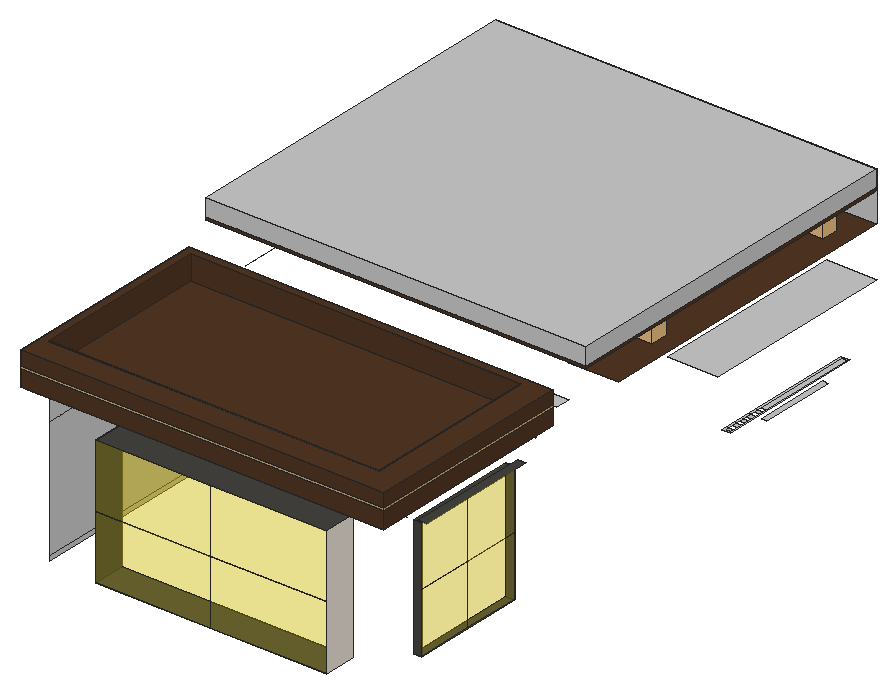
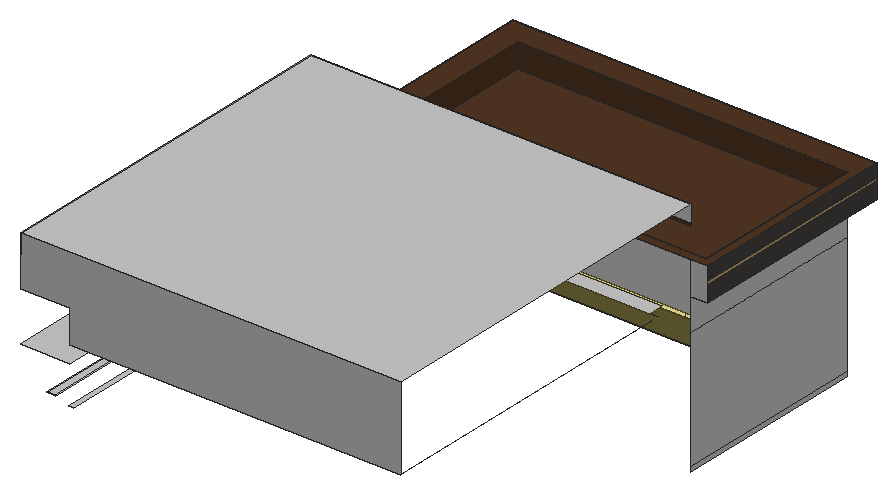
# SketchUp Ruby script. Lengths in inches.
U = 1.inch
M = Sketchup.active_model
def pt(a) = Geom::Point3d.new(a.map { |v| v * U })
def face(e, loops, mat)
  f = e.add_face(loops[0].map { |a| pt(a) })
  loops[1..].each { |l| e.add_face(l.map { |a| pt(a) }).erase! }
  f.material = f.back_material = mat if mat
  f
end
# faces: each face lists its corners as indices into pts; further lists are holes
def faces(e, pts, list, mat = nil) = list.each { |f| face(e, (f[0].is_a?(Array) ? f : [f]).map { |l| l.map { |i| pts[i] } }, mat) }
# xy, xz, yz: faces in a plane at the given z, y or x. An outline is a flat list of corners, or four numbers for a rectangle; further outlines are holes
def ring(l) = l.size == 4 ? [[l[0], l[1]], [l[2], l[1]], [l[2], l[3]], [l[0], l[3]]] : l.each_slice(2).to_a
def flat(e, list, mat, &to3) = list.each { |f| face(e, (f[0].is_a?(Array) ? f : [f]).map { |l| ring(l).map { |u, v| to3.(u, v) } }, mat) }
def xy(e, z, list, mat = nil) = flat(e, list, mat) { |x, y| [x, y, z] }
def xz(e, y, list, mat = nil) = flat(e, list, mat) { |x, z| [x, y, z] }
def yz(e, x, list, mat = nil) = flat(e, list, mat) { |y, z| [x, y, z] }
def lines(e, pts, list) = list.each { |a, b| e.add_line(pt(pts[a]), pt(pts[b])) }
# prism: a flat outline (further loops are holes) pulled along v
def prism(e, loops, v, mat = nil)
  f = face(e, loops, mat); d = Geom::Vector3d.new(v.map { |x| x * U })
  f.pushpull(f.normal.samedirection?(d) ? d.length : -d.length)
end
def box(e, o, s, mat = nil) = prism(e, [[o, [o[0] + s[0], o[1], o[2]], [o[0] + s[0], o[1] + s[1], o[2]], [o[0], o[1] + s[1], o[2]]]], [0, 0, s[2]], mat)
def at(x, y, z, deg = 0) = Geom::Transformation.translation(pt([x, y, z])) * Geom::Transformation.rotation(ORIGIN, Z_AXIS, deg.degrees)
def axes(o, x, y, z) = Geom::Transformation.new([*x, 0, *y, 0, *z, 0, *pt(o).to_a, 1])
def part(name) = M.definitions.add(name)
# library, detail: a bought-in or finely detailed component or shape, given as its bounding box
def library(name, o, s) = part(name).tap { |d| box(d.entities, o, s) }
def detail(e, o, s) = box(e.add_group.entities, o, s)
def put(e, d, t, mat = nil) = e.add_instance(d, t).tap { |i| i.material = mat if mat }
def group(e, t, mat = nil) = e.add_group.tap { |g| g.transformation = t; g.material = mat if mat }.entities
root = M.entities
M.materials.add("Glass_Basic_01").color = [255, 228, 0]
M.materials["Glass_Basic_01"].alpha = 0.25
M.materials.add("Marble_01_1K").color = [230, 221, 211]
M.materials.add("Plywood_08_1K").color = [202, 166, 113]
M.materials.add("Wood_Planks_01_1K").color = [69, 67, 63]
M.materials.add("Wood_Veneer_15_1K").color = [81, 54, 35]
M.materials.add("[_0053_Ivory_]").color = [200, 200, 200]
c1 = library("Sphere Light\#3",[-4.91,-4.91,-4.91],[9.82,9.82,9.82])
c2 = library("Sphere Light\#2",[-4.71,-4.71,-4.71],[9.42,9.42,9.42])
c3 = library("Sphere Light\#1",[-6.34,-6.34,-6.34],[12.68,12.68,12.68])
c4 = library("Sphere Light",[-6.24,-6.24,-6.24],[12.48,12.48,12.48])
xy(root,267,[[410.51,98.15,578.51,122.15]],"Wood_Planks_01_1K")
xy(root,270,[[605.51,143.15,611.51,227.15]],"Wood_Planks_01_1K")
xy(root,318,[[643.1,411.95,647.1,467.15]],"[_0053_Ivory_]")
xy(root,330,[[[647.1,371.15,653.51,479.15],[648.1,372.15,652.51,478.15]],[648.1,372.15,652.51,375.42],[648.1,378.69,652.51,381.96],[648.1,385.24,652.51,388.51],[648.1,391.78,652.51,395.05],
  [648.1,398.33,652.51,401.6],[648.1,404.87,652.51,478.15]],"[_0053_Ivory_]")
xy(root,357,[[605.51,143.15,611.51,227.15]],"Wood_Planks_01_1K")
xy(root,360,[[410.51,98.15,578.51,122.15],[611.51,140.15,617.51,230.15]],"Wood_Planks_01_1K")
xy(root,372,[[386.51,122.15,605.51,239.15],[617.51,359.15,653.51,503.15]],"[_0053_Ivory_]")
xy(root,384,[[365.51,98.15,365.51,239.15,377.51,239.15,377.51,98.15,377.33,98.15,376.79,98.5625,375.34,99.16,373.79,99.37,372.23,99.16,370.79,98.5625,370.25,98.15]],"Wood_Planks_01_1K")
xy(root,384,[[365.51,86.15,365.51,98.15,370.25,98.15,369.55,97.61,368.59,96.37,367.99,94.92,367.79,93.37,367.99,91.8125,368.59,90.37,369.55,89.12,370.79,88.17,372.23,87.57,373.79,87.37,375.34,87.57,376.79,88.17,378.03,89.12,378.98,90.37,379.58,91.8125,379.79,93.37,379.58,94.92,378.98,96.37,378.03,97.61,377.33,98.15,618.11,98.15,617.41,97.61,616.46,96.37,615.86,94.92,615.65,93.37,615.86,91.8125,616.46,90.37,617.41,89.12,618.65,88.17,620.1,87.57,621.65,87.37,623.2,87.57,624.65,88.17,625.89,89.12,626.85,90.37,627.45,91.8125,627.65,93.37,627.45,94.92,626.85,96.37,625.89,97.61,625.19,98.15,629.51,98.15,629.51,86.15],[617.51,98.15,617.51,239.15,629.51,239.15,629.51,98.15,625.19,98.15,624.65,98.5625,623.2,99.16,621.65,99.37,620.1,99.16,618.65,98.5625,618.11,98.15]],"Wood_Veneer_15_1K")
xy(root,384,[[383.51,257.92,617.51,269.15]],"[_0053_Ivory_]")
xy(root,387,[[373.79,87.37,372.23,87.57,370.79,88.17,369.55,89.12,368.59,90.37,367.99,91.8125,367.79,93.37,367.99,94.92,368.59,96.37,369.55,97.61,370.25,98.15,370.79,98.5625,372.23,99.16,373.79,99.37,375.34,99.16,376.79,98.5625,377.33,98.15,378.03,97.61,378.98,96.37,379.58,94.92,379.79,93.37,379.58,91.8125,378.98,90.37,378.03,89.12,376.79,88.17,375.34,87.57],[621.65,87.37,620.1,87.57,618.65,88.17,617.41,89.12,616.46,90.37,615.86,91.8125,615.65,93.37,615.86,94.92,616.46,96.37,617.41,97.61,618.11,98.15,618.65,98.5625,620.1,99.16,621.65,99.37,623.2,99.16,624.65,98.5625,625.19,98.15,625.89,97.61,626.85,96.37,627.45,94.92,627.65,93.37,627.45,91.8125,626.85,90.37,625.89,89.12,624.65,88.17,623.2,87.57]],"Wood_Veneer_15_1K")
xy(root,390.44,[[371.51,104.15,611.51,233.15]],"Wood_Veneer_15_1K")
xy(root,408,[[[365.51,86.15,629.51,239.15],[371.51,104.15,611.51,233.15]],[[617.51,269.15,653.51,503.15],[633.43,316.8125,634.98,317.02,636.43,317.62,637.67,318.57,638.62,319.8125,639.22,321.26,639.43,322.8125,639.22,324.37,638.62,325.8125,637.67,327.06,636.43,328.01,634.98,328.61,633.43,328.8125,631.875,328.61,630.43,328.01,629.18,327.06,628.23,325.8125,627.63,324.37,627.43,322.8125,627.63,321.26,628.23,319.8125,629.18,318.57,630.43,317.62,631.875,317.02],[633.43,471.47,634.98,471.67,636.43,472.27,637.67,473.23,638.62,474.47,639.22,475.92,639.43,477.47,639.22,479.02,638.62,480.47,637.67,481.71,636.43,482.66,634.98,483.26,633.43,483.47,631.875,483.26,630.43,482.66,629.18,481.71,628.23,480.47,627.63,479.02,627.43,477.47,627.63,475.92,628.23,474.47,629.18,473.23,630.43,472.27,631.875,471.67]]],"Wood_Veneer_15_1K")
xy(root,411,[[633.43,316.8125,631.875,317.02,630.43,317.62,629.18,318.57,628.23,319.8125,627.63,321.26,627.43,322.8125,627.63,324.37,628.23,325.8125,629.18,327.06,630.43,328.01,631.875,328.61,633.43,328.8125,634.98,328.61,636.43,328.01,637.67,327.06,638.62,325.8125,639.22,324.37,639.43,322.8125,639.22,321.26,638.62,319.8125,637.67,318.57,636.43,317.62,634.98,317.02],[633.43,471.47,631.875,471.67,630.43,472.27,629.18,473.23,628.23,474.47,627.63,475.92,627.43,477.47,627.63,479.02,628.23,480.47,629.18,481.71,630.43,482.66,631.875,483.26,633.43,483.47,634.98,483.26,636.43,482.66,637.67,481.71,638.62,480.47,639.22,479.02,639.43,477.47,639.22,475.92,638.62,474.47,637.67,473.23,636.43,472.27,634.98,471.67]],"Wood_Veneer_15_1K")
xy(root,444,[[377.51,239.15,653.51,503.15]],"[_0053_Ivory_]")
xz(root,86.15,[[365.51,396,629.51,398]],"Plywood_08_1K")
xz(root,86.15,[[365.51,384,629.51,396],[365.51,398,629.51,408]],"Wood_Veneer_15_1K")
xz(root,98.15,[[410.51,267,494.51,313.5],[494.51,267,578.51,313.5],[410.51,313.5,494.51,360],[494.51,313.5,578.51,360]],"Glass_Basic_01")
xz(root,104.15,[[371.51,390.44,611.51,408]],"Wood_Veneer_15_1K")
xz(root,122.15,[[410.51,267,578.51,360]],"Glass_Basic_01")
xz(root,143.15,[[605.51,270,611.51,357]],"Wood_Planks_01_1K")
xz(root,227.15,[[605.51,270,611.51,357]],"Wood_Planks_01_1K")
xz(root,233.15,[[371.51,390.44,611.51,408]],"Wood_Veneer_15_1K")
xz(root,239.15,[[377.51,430,653.51,432]],"Wood_Veneer_15_1K")
xz(root,239.15,[[377.51,372,617.51,372,617.51,384,629.51,384,629.51,408,377.51,408],[365.51,384,377.51,408],[377.51,432,653.51,444]],"[_0053_Ivory_]")
xz(root,503.15,[[377.51,384,377.51,444,653.51,444,653.51,408,617.51,408,617.51,384]],"[_0053_Ivory_]")
yz(root,365.51,[[86.15,396,239.15,398]],"Plywood_08_1K")
yz(root,365.51,[[86.15,384,239.15,396],[86.15,398,239.15,408]],"Wood_Planks_01_1K")
yz(root,371.51,[[104.15,390.44,233.15,408]],"Wood_Veneer_15_1K")
yz(root,377.51,[[98.15,270,239.15,273],[98.15,273,239.15,360],[98.15,360,239.15,384]],"[_0053_Ivory_]")
yz(root,410.51,[[98.15,267,122.15,360]],"Wood_Planks_01_1K")
yz(root,578.51,[[98.15,267,122.15,360]],"Marble_01_1K")
yz(root,605.51,[[143.15,270,227.15,357]],"Glass_Basic_01")
yz(root,611.51,[[143.15,270,185.15,313.5],[185.15,270,227.15,313.5],[143.15,313.5,185.15,357],[185.15,313.5,227.15,357]],"Glass_Basic_01")
yz(root,611.51,[[104.15,390.44,233.15,408]],"Wood_Veneer_15_1K")
yz(root,629.51,[[86.15,396,239.15,398]],"Plywood_08_1K")
yz(root,629.51,[[86.15,384,239.15,396],[86.15,398,239.15,408]],"Wood_Veneer_15_1K")
yz(root,653.51,[[239.15,430,503.15,432]],"Wood_Veneer_15_1K")
yz(root,653.51,[[239.15,432,503.15,444]],"[_0053_Ivory_]")
p = [[373.79,87.37,384],[372.23,87.57,384],[372.23,87.57,387],[373.79,87.37,387],[375.34,87.57,384],[375.34,87.57,387],
  [621.65,87.37,384],[620.1,87.57,384],[620.1,87.57,387],[621.65,87.37,387],[623.2,87.57,384],[623.2,87.57,387],
  [370.79,88.17,384],[370.79,88.17,387],[376.79,88.17,384],[376.79,88.17,387],[618.65,88.17,384],[618.65,88.17,387],
  [624.65,88.17,384],[624.65,88.17,387],[369.55,89.12,384],[369.55,89.12,387],[378.03,89.12,384],[378.03,89.12,387],
  [617.41,89.12,384],[617.41,89.12,387],[625.89,89.12,384],[625.89,89.12,387],[368.59,90.37,384],[368.59,90.37,387],
  [378.98,90.37,384],[378.98,90.37,387],[616.46,90.37,384],[616.46,90.37,387],[626.85,90.37,384],[626.85,90.37,387],
  [367.99,91.8125,384],[367.99,91.8125,387],[379.58,91.8125,384],[379.58,91.8125,387],[615.86,91.8125,384],[615.86,91.8125,387],
  [627.45,91.8125,384],[627.45,91.8125,387],[367.79,93.37,384],[367.79,93.37,387],[379.79,93.37,384],[379.79,93.37,387],
  [615.65,93.37,384],[615.65,93.37,387],[627.65,93.37,384],[627.65,93.37,387],[367.99,94.92,384],[367.99,94.92,387],
  [379.58,94.92,384],[379.58,94.92,387],[615.86,94.92,384],[615.86,94.92,387],[627.45,94.92,384],[627.45,94.92,387],
  [368.59,96.37,384],[368.59,96.37,387],[378.98,96.37,384],[378.98,96.37,387],[616.46,96.37,384],[616.46,96.37,387],
  [626.85,96.37,384],[626.85,96.37,387],[369.55,97.61,384],[369.55,97.61,387],[378.03,97.61,384],[378.03,97.61,387],
  [617.41,97.61,384],[617.41,97.61,387],[625.89,97.61,384],[625.89,97.61,387],[370.25,98.15,384],[370.25,98.15,387],
  [377.33,98.15,384],[377.33,98.15,387],[618.11,98.15,384],[618.11,98.15,387],[625.19,98.15,384],[625.19,98.15,387],
  [370.79,98.5625,384],[370.79,98.5625,387],[376.79,98.5625,384],[376.79,98.5625,387],[618.65,98.5625,384],[618.65,98.5625,387],
  [624.65,98.5625,384],[624.65,98.5625,387],[372.23,99.16,384],[372.23,99.16,387],[375.34,99.16,384],[375.34,99.16,387],
  [620.1,99.16,384],[620.1,99.16,387],[623.2,99.16,384],[623.2,99.16,387],[373.79,99.37,384],[373.79,99.37,387],
  [621.65,99.37,384],[621.65,99.37,387],[633.43,316.8125,408],[631.875,317.02,408],[631.875,317.02,411],[633.43,316.8125,411],
  [634.98,317.02,408],[634.98,317.02,411],[630.43,317.62,408],[630.43,317.62,411],[636.43,317.62,408],[636.43,317.62,411],
  [629.18,318.57,408],[629.18,318.57,411],[637.67,318.57,408],[637.67,318.57,411],[628.23,319.8125,408],[628.23,319.8125,411],
  [638.62,319.8125,408],[638.62,319.8125,411],[627.63,321.26,408],[627.63,321.26,411],[639.22,321.26,408],[639.22,321.26,411],
  [627.43,322.8125,408],[627.43,322.8125,411],[639.43,322.8125,408],[639.43,322.8125,411],[627.63,324.37,408],[627.63,324.37,411],
  [639.22,324.37,408],[639.22,324.37,411],[628.23,325.8125,408],[628.23,325.8125,411],[638.62,325.8125,408],[638.62,325.8125,411],
  [629.18,327.06,408],[629.18,327.06,411],[637.67,327.06,408],[637.67,327.06,411],[630.43,328.01,408],[630.43,328.01,411],
  [636.43,328.01,408],[636.43,328.01,411],[631.875,328.61,408],[631.875,328.61,411],[634.98,328.61,408],[634.98,328.61,411],
  [633.43,328.8125,408],[633.43,328.8125,411],[633.43,471.47,408],[631.875,471.67,408],[631.875,471.67,411],[633.43,471.47,411],
  [634.98,471.67,408],[634.98,471.67,411],[630.43,472.27,408],[630.43,472.27,411],[636.43,472.27,408],[636.43,472.27,411],
  [629.18,473.23,408],[629.18,473.23,411],[637.67,473.23,408],[637.67,473.23,411],[628.23,474.47,408],[628.23,474.47,411],
  [638.62,474.47,408],[638.62,474.47,411],[627.63,475.92,408],[627.63,475.92,411],[639.22,475.92,408],[639.22,475.92,411],
  [627.43,477.47,408],[627.43,477.47,411],[639.43,477.47,408],[639.43,477.47,411],[627.63,479.02,408],[627.63,479.02,411],
  [639.22,479.02,408],[639.22,479.02,411],[628.23,480.47,408],[628.23,480.47,411],[638.62,480.47,408],[638.62,480.47,411],
  [629.18,481.71,408],[629.18,481.71,411],[637.67,481.71,408],[637.67,481.71,411],[630.43,482.66,408],[630.43,482.66,411],
  [636.43,482.66,408],[636.43,482.66,411],[631.875,483.26,408],[631.875,483.26,411],[634.98,483.26,408],[634.98,483.26,411],
  [633.43,483.47,408],[633.43,483.47,411],[383.51,269.15,384],[377.51,269.15,384],[377.51,275.15,384],[377.51,503.15,384],
  [386.51,122.15,372],[386.51,110.15,372],[605.51,122.15,372],[617.51,122.15,372]]
faces(root,p,[[0,1,2,3],[4,0,3,5],[6,7,8,9],[10,6,9,11],[1,12,13,2],[14,4,5,15],[7,16,17,8],[18,10,11,19],
  [12,20,21,13],[22,14,15,23],[16,24,25,17],[26,18,19,27],[20,28,29,21],[30,22,23,31],[24,32,33,25],[34,26,27,35],
  [28,36,37,29],[38,30,31,39],[32,40,41,33],[42,34,35,43],[36,44,45,37],[46,38,39,47],[40,48,49,41],[50,42,43,51],
  [44,52,53,45],[54,46,47,55],[48,56,57,49],[58,50,51,59],[52,60,61,53],[62,54,55,63],[56,64,65,57],[66,58,59,67],
  [60,68,69,61],[70,62,63,71],[64,72,73,65],[74,66,67,75],[68,76,77,69],[78,70,71,79],[72,80,81,73],[82,74,75,83],
  [76,84,85,77],[86,78,79,87],[80,88,89,81],[90,82,83,91],[84,92,93,85],[94,86,87,95],[88,96,97,89],[98,90,91,99],
  [92,100,101,93],[100,94,95,101],[96,102,103,97],[102,98,99,103],[104,105,106,107],[108,104,107,109],[105,110,111,106],[112,108,109,113],
  [110,114,115,111],[116,112,113,117],[114,118,119,115],[120,116,117,121],[118,122,123,119],[124,120,121,125],[122,126,127,123],[128,124,125,129],
  [126,130,131,127],[132,128,129,133],[130,134,135,131],[136,132,133,137],[134,138,139,135],[140,136,137,141],[138,142,143,139],[144,140,141,145],
  [142,146,147,143],[148,144,145,149],[146,150,151,147],[150,148,149,151],[152,153,154,155],[156,152,155,157],[153,158,159,154],[160,156,157,161],
  [158,162,163,159],[164,160,161,165],[162,166,167,163],[168,164,165,169],[166,170,171,167],[172,168,169,173],[170,174,175,171],[176,172,173,177],
  [174,178,179,175],[180,176,177,181],[178,182,183,179],[184,180,181,185],[182,186,187,183],[188,184,185,189],[186,190,191,187],[192,188,189,193],
  [190,194,195,191],[196,192,193,197],[194,198,199,195],[198,196,197,199]],"Wood_Veneer_15_1K")
lines(root,p,[[200,201],[202,203],[204,205],[206,207]])
put(root,c1,at(373.62,93.55,387),"[_0053_Ivory_]")
put(root,c2,at(621.19,93.42,387),"[_0053_Ivory_]")
put(root,c3,at(633.73,322.11,411),"[_0053_Ivory_]")
put(root,c4,at(633.67,477.43,411),"[_0053_Ivory_]")
